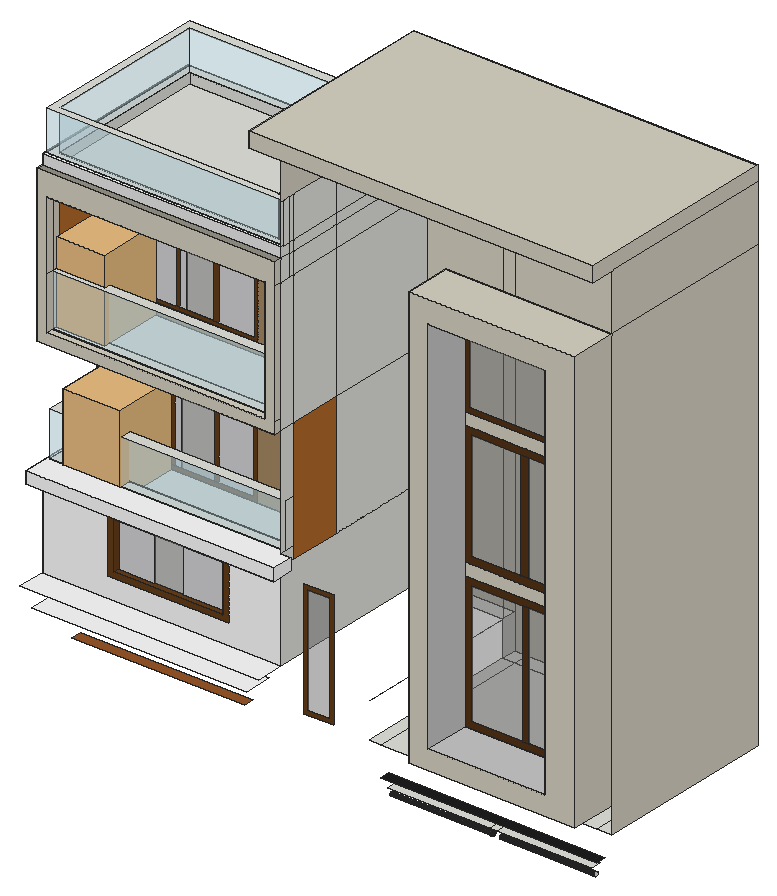
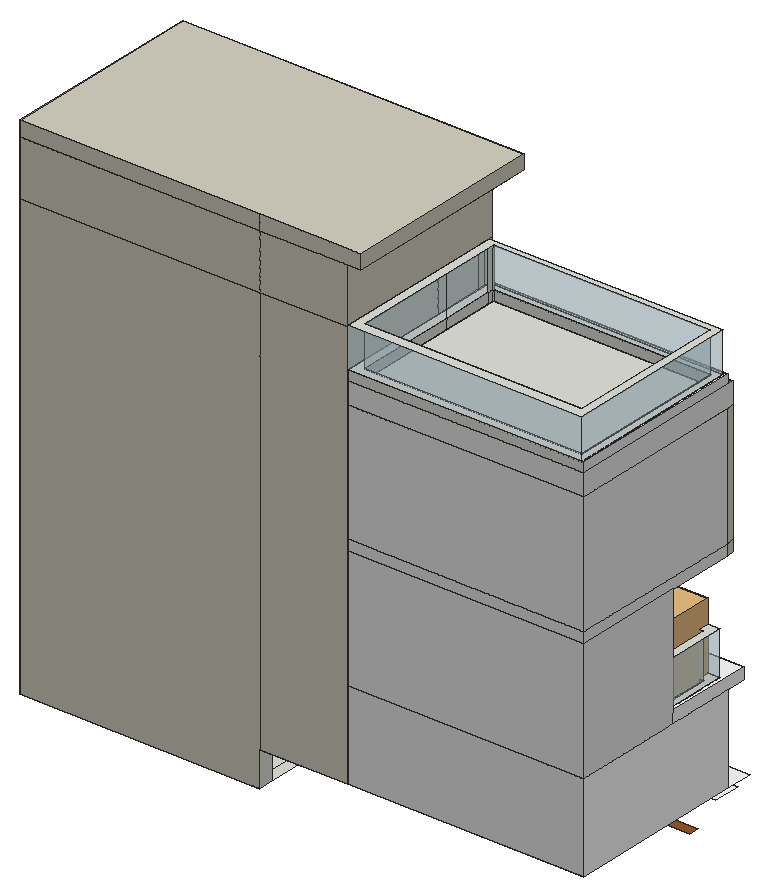
# SketchUp Ruby script. Lengths in inches.
U = 1.inch
M = Sketchup.active_model
def pt(a) = Geom::Point3d.new(a.map { |v| v * U })
def face(e, loops, mat)
  f = e.add_face(loops[0].map { |a| pt(a) })
  loops[1..].each { |l| e.add_face(l.map { |a| pt(a) }).erase! }
  f.material = f.back_material = mat if mat
  f
end
# faces: each face lists its corners as indices into pts; further lists are holes
def faces(e, pts, list, mat = nil) = list.each { |f| face(e, (f[0].is_a?(Array) ? f : [f]).map { |l| l.map { |i| pts[i] } }, mat) }
# xy, xz, yz: faces in a plane at the given z, y or x. An outline is a flat list of corners, or four numbers for a rectangle; further outlines are holes
def ring(l) = l.size == 4 ? [[l[0], l[1]], [l[2], l[1]], [l[2], l[3]], [l[0], l[3]]] : l.each_slice(2).to_a
def flat(e, list, mat, &to3) = list.each { |f| face(e, (f[0].is_a?(Array) ? f : [f]).map { |l| ring(l).map { |u, v| to3.(u, v) } }, mat) }
def xy(e, z, list, mat = nil) = flat(e, list, mat) { |x, y| [x, y, z] }
def xz(e, y, list, mat = nil) = flat(e, list, mat) { |x, z| [x, y, z] }
def yz(e, x, list, mat = nil) = flat(e, list, mat) { |y, z| [x, y, z] }
def lines(e, pts, list) = list.each { |a, b| e.add_line(pt(pts[a]), pt(pts[b])) }
# prism: a flat outline (further loops are holes) pulled along v
def prism(e, loops, v, mat = nil)
  f = face(e, loops, mat); d = Geom::Vector3d.new(v.map { |x| x * U })
  f.pushpull(f.normal.samedirection?(d) ? d.length : -d.length)
end
def box(e, o, s, mat = nil) = prism(e, [[o, [o[0] + s[0], o[1], o[2]], [o[0] + s[0], o[1] + s[1], o[2]], [o[0], o[1] + s[1], o[2]]]], [0, 0, s[2]], mat)
def at(x, y, z, deg = 0) = Geom::Transformation.translation(pt([x, y, z])) * Geom::Transformation.rotation(ORIGIN, Z_AXIS, deg.degrees)
def axes(o, x, y, z) = Geom::Transformation.new([*x, 0, *y, 0, *z, 0, *pt(o).to_a, 1])
def part(name) = M.definitions.add(name)
# library, detail: a bought-in or finely detailed component or shape, given as its bounding box
def library(name, o, s) = part(name).tap { |d| box(d.entities, o, s) }
def detail(e, o, s) = box(e.add_group.entities, o, s)
def put(e, d, t, mat = nil) = e.add_instance(d, t).tap { |i| i.material = mat if mat }
def group(e, t, mat = nil) = e.add_group.tap { |g| g.transformation = t; g.material = mat if mat }.entities
root = M.entities
M.materials.add("[Blinds Vertical Pattern]").color = [212, 212, 214]
M.materials.add("[Blinds Weave]").color = [141, 91, 25]
M.materials.add("[Carrera Marble]").color = [252, 252, 252]
M.materials.add("[Carrera Marble]1").color = [234, 234, 234]
M.materials.add("[Color M02]").color = [198, 198, 198]
M.materials.add("[Color M07]").color = [58, 58, 58]
M.materials.add("[Color M08]").color = [30, 30, 30]
M.materials.add("[Formica Graystone]").color = [214, 209, 194]
M.materials.add("[Formica Graystone]1").color = [149, 146, 135]
M.materials.add("[Quartz Light Grey]").color = [251, 251, 252]
M.materials.add("[Translucent Glass Gray]").color = [128, 128, 128]
M.materials["[Translucent Glass Gray]"].alpha = 0.5
M.materials.add("[Translucent Glass Safety]").color = [213, 245, 255]
M.materials["[Translucent Glass Safety]"].alpha = 0.35
M.materials.add("[Wallpaper Stripe]").color = [165, 138, 99]
M.materials.add("[Wood Bamboo]").color = [177, 105, 43]
M.materials.add("[Wood Cherry Original]").color = [152, 86, 42]
M.materials.add("[Wood Floor Dark]").color = [84, 51, 23]
M.materials.add("[Wood Floor Parquet]").color = [102, 62, 27]
M.materials.add("[Wood Floor Parquet]1").color = [145, 89, 39]
c1 = library("chau cay",[-24.34,-109.24,0],[56.46,62.58,79.69])
xy(root,113.6,[[473.77,406.29,574.36,416.16],[574.36,406.29,581.54,416.16],[581.54,406.29,674.94,416.16]])
xy(root,119.75,[[467.61,406.29,674.94,416.16],[674.94,406.29,679.23,416.16]],"[Color M08]")
xy(root,136.93,[[163.95,406.29,333.85,416.16]],"[Wood Cherry Original]")
xy(root,149.125,[[456.06,406.29,467.61,570.65],[467.61,406.29,679.23,570.65],[679.23,406.29,694.52,585.18],[456.06,570.65,467.61,585.18],[467.61,570.65,679.23,585.18]])
xy(root,168.73,[[146.33,378.85,357.05,406.29]],"[Carrera Marble]")
xy(root,175.14,[[531.06,361.1,694.52,406.29]],"[Formica Graystone]")
xy(root,183.6875,[[134.55,406.29,369,570.65],[134.55,570.65,369,585.18],[369,570.65,456.06,585.18]])
xy(root,183.6875,[[134.55,378.85,369,406.29]],"[Carrera Marble]")
xy(root,194.17,[[550.09,361.1,664.36,406.29]],"[Color M02]")
xy(root,208.41,[[204.29,406.29,312.26,412.54]],"[Wood Floor Parquet]")
xy(root,255.64,[[204.29,406.29,312.26,412.54]],"[Wood Floor Parquet]")
xy(root,270.8125,[[134.55,406.29,134.55,473.7,145.55,473.7,145.55,422.06,369,422.06,369,406.29],[145.55,422.06,369,473.7],[134.55,473.7,369,585.18]])
xy(root,270.8125,[[134.55,385.54,378.87,406.29]],"[Wood Bamboo]")
xy(root,276.39,[[320.76,473.7,360.82,482.32]],"[Wood Floor Parquet]1")
xy(root,282.625,[[137.78,411.51,137.78,473.7,145.55,473.7,145.55,422.06,369,422.06,369,411.51]])
xy(root,282.625,[[134.55,385.54,378.87,385.54,378.87,406.29,369,406.29,369,411.51,137.78,411.51,137.78,473.7,134.55,473.7]],"[Carrera Marble]")
xy(root,326.4375,[[137.78,411.51,369,411.51,369,422.06,145.55,422.06,145.55,473.7,137.78,473.7]])
xy(root,353.33,[[320.76,473.7,360.82,482.32]],"[Wood Floor Parquet]1")
xy(root,390.8125,[[134.55,406.29,145.55,473.7],[145.55,406.29,369,473.7],[134.55,473.7,369,585.18]])
xy(root,390.8125,[[134.55,399.16,145.55,406.29],[145.55,399.16,369,406.29]],"[Formica Graystone]")
xy(root,401.5,[[144.33,406.29,359.22,416.07],[144.33,416.07,359.22,473.7],[144.33,473.7,359.22,575.4]])
xy(root,401.5,[[144.33,399.16,359.22,406.29]],"[Formica Graystone]")
xy(root,416.25,[[308.63,473.7,346.63,482.95]])
xy(root,453.125,[[144.33,406.29,359.22,416.07]])
xy(root,483.25,[[308.63,473.7,346.63,482.95]],"[Wood Floor Parquet]1")
xy(root,521.5,[[134.55,406.29,144.33,416.07],[359.22,406.29,369,416.07],[134.55,416.07,144.33,473.7],[359.22,416.07,369,422.06],[359.22,422.06,369,473.7],
  [134.55,473.7,144.33,585.18],[144.33,473.7,359.22,575.4],[359.22,473.7,369,585.18],[144.33,575.4,359.22,585.18]])
xy(root,521.5,[[144.33,399.16,359.22,473.7]],"[Wood Bamboo]")
xy(root,542.8125,[[[134.55,406.29,369,585.18],[143.9,415.64,359.65,575.83]],[143.9,415.64,359.65,575.83]])
xy(root,542.8125,[[134.55,399.16,369,406.29]],"[Formica Graystone]1")
xy(root,552.5,[[[136.62,409.6,369,585.18],[143.9,415.64,359.65,575.83]]])
xy(root,552.5,[[134.55,406.29,369,409.6],[134.55,409.6,136.62,585.18]],"[Quartz Light Grey]")
xy(root,568.18,[[550.09,361.1,664.36,406.29]],"[Color M02]")
xy(root,590.25,[[531.06,361.1,694.52,406.29]],"[Formica Graystone]")
xy(root,592.1875,[[[136.62,409.6,369,585.18],[143.9,415.64,359.65,575.83]]])
xy(root,645.75,[[369,406.29,694.52,585.18]])
xy(root,645.75,[[356.12,382.85,694.52,406.29],[356.12,406.29,369,585.18]],"[Formica Graystone]")
xy(root,660.4375,[[356.12,382.85,694.52,585.18]],"[Formica Graystone]")
xz(root,361.1,[[[531.06,175.14,694.52,590.25],[550.09,194.17,664.36,568.18]]],"[Formica Graystone]")
xz(root,382.85,[[356.12,645.75,694.52,660.4375]],"[Formica Graystone]")
xz(root,385.54,[[134.55,270.8125,378.87,282.625]],"[Carrera Marble]")
xz(root,399.16,[[[134.55,390.8125,369,542.8125],[144.33,401.5,359.22,521.5]]],"[Formica Graystone]")
xz(root,406.29,[[[531.06,175.14,694.52,590.25],[550.09,194.17,664.36,568.18]],[369,270.8125,378.87,282.625],[134.55,390.8125,134.55,521.5,144.33,521.5,144.33,401.5,359.22,401.5,359.22,521.5,369,521.5,369,390.8125]])
xz(root,406.29,[[[134.55,183.6875,369,270.8125],[199.09,203.21,317.46,260.84]]],"[Carrera Marble]")
xz(root,406.29,[[134.55,542.8125,369,552.5]],"[Carrera Marble]1")
xz(root,406.29,[[550.09,326.9,664.36,339.04],[550.09,459.62,664.36,471.47]],"[Formica Graystone]")
xz(root,406.29,[[395.5625,153.71,416.96,260.54],[556.47,200.55,606.76,320.52],[612.79,200.55,657.99,320.52],[556.8,345.75,604.91,452.91],[612.27,345.75,657.65,452.91],
  [555.11,476.49,659.35,563.16]],"[Translucent Glass Gray]")
xz(root,406.29,[[144.33,401.5,359.22,453.125]],"[Translucent Glass Safety]")
xz(root,406.29,[[[550.09,194.17,664.36,326.9],[556.47,200.55,657.99,320.52]],[606.76,200.55,612.79,320.52],[[550.09,339.04,664.36,459.62],[556.8,345.75,657.65,452.91]],[604.91,345.75,612.27,452.91],[[550.09,471.47,664.36,568.18],[555.11,476.49,659.35,563.16]]],"[Wood Floor Dark]")
xz(root,406.29,[[[391.83,149.97,420.7,264.27],[395.5625,153.71,416.96,260.54]],[[199.09,203.21,317.46,260.84],[204.29,208.41,312.26,255.64]]],"[Wood Floor Parquet]")
xz(root,409.6,[[136.62,552.5,369,592.1875]],"[Translucent Glass Safety]")
xz(root,411.51,[[137.78,282.625,369,326.4375]],"[Translucent Glass Safety]")
xz(root,412.54,[[204.29,208.41,240,255.64],[268.36,208.41,312.26,255.64]],"[Blinds Vertical Pattern]")
xz(root,412.54,[[240,208.41,268.36,255.64]],"[Translucent Glass Gray]")
xz(root,415.64,[[143.9,542.8125,359.65,552.5]])
xz(root,415.64,[[143.9,552.5,359.65,592.1875]],"[Translucent Glass Safety]")
xz(root,416.07,[[144.33,401.5,359.22,453.125]],"[Translucent Glass Safety]")
xz(root,422.06,[[145.55,270.8125,369,282.625]])
xz(root,422.06,[[145.55,282.625,369,326.4375]],"[Translucent Glass Safety]")
xz(root,473.7,[[134.55,270.8125,145.55,282.625],[134.55,282.625,137.78,282.625,137.78,326.4375,145.55,326.4375,145.55,390.8125,134.55,390.8125],[137.78,282.625,145.55,326.4375]])
xz(root,473.7,[[175.44,274.72,207.12,374.1],[210.96,274.72,218.06,374.1],[254.34,274.72,288.69,374.1],[174.75,416.21,211.53,501.07],[216.17,416.21,223.04,501.07],
  [254.11,416.21,288.86,501.07]],"[Blinds Vertical Pattern]")
xz(root,473.7,[[218.06,274.72,250.5,374.1],[223.04,416.21,249.47,501.07]],"[Translucent Glass Gray]")
xz(root,473.7,[[[145.55,270.8125,171.54,270.8125,171.54,378,292.6,378,292.6,270.8125,369,270.8125,369,390.8125,145.55,390.8125],[320.76,276.39,360.82,353.33]],[[144.33,401.5,359.22,521.5],[170.84,412.3,292.77,504.98],[308.63,416.25,346.63,483.25]]],"[Wallpaper Stripe]")
xz(root,473.7,[[[171.54,270.8125,292.6,378],[175.44,274.72,288.69,374.1]],[207.12,274.72,210.96,374.1],[250.5,274.72,254.34,374.1],[[170.84,412.3,292.77,504.98],[174.75,416.21,288.86,501.07]],[211.53,416.21,216.17,501.07],
  [249.47,416.21,254.11,501.07]],"[Wood Floor Parquet]")
xz(root,482.32,[[320.76,276.39,360.82,353.33]],"[Blinds Weave]")
xz(root,482.95,[[308.63,416.25,346.63,483.25]],"[Blinds Weave]")
xz(root,575.4,[[144.33,401.5,359.22,521.5]])
xz(root,575.83,[[143.9,542.8125,359.65,552.5]])
xz(root,575.83,[[143.9,552.5,359.65,592.1875]],"[Translucent Glass Safety]")
xz(root,585.18,[[134.55,542.8125,369,552.5]])
xz(root,585.18,[[134.55,183.6875,369,270.8125],[134.55,270.8125,369,390.8125],[134.55,390.8125,369,401.5],[134.55,401.5,369,521.5],[134.55,521.5,369,542.8125]],"[Carrera Marble]1")
xz(root,585.18,[[456.06,149.125,694.52,590.25],[369,183.6875,456.06,590.25],[369,590.25,456.06,645.75],[456.06,590.25,694.52,645.75],[356.12,645.75,456.06,660.4375],
  [456.06,645.75,694.52,660.4375]],"[Formica Graystone]")
xz(root,585.18,[[136.62,552.5,369,592.1875]],"[Translucent Glass Safety]")
yz(root,134.55,[[406.29,183.6875,585.18,270.8125],[385.54,270.8125,473.7,282.625]],"[Carrera Marble]")
yz(root,134.55,[[473.7,270.8125,585.18,390.8125],[406.29,390.8125,585.18,401.5],[406.29,401.5,585.18,521.5],[399.16,521.5,585.18,542.8125],[406.29,542.8125,585.18,552.5]],"[Carrera Marble]1")
yz(root,134.55,[[399.16,390.8125,406.29,401.5],[399.16,401.5,406.29,521.5]],"[Formica Graystone]")
yz(root,136.62,[[409.6,552.5,585.18,592.1875]],"[Translucent Glass Safety]")
yz(root,137.78,[[411.51,282.625,473.7,326.4375]],"[Translucent Glass Safety]")
yz(root,143.9,[[415.64,542.8125,575.83,552.5]])
yz(root,143.9,[[415.64,552.5,575.83,592.1875]],"[Translucent Glass Safety]")
yz(root,144.33,[[406.29,401.5,416.07,453.125],[473.7,401.5,575.4,521.5]])
yz(root,144.33,[[399.16,401.5,406.29,453.125],[399.16,453.125,406.29,521.5],[406.29,453.125,416.07,521.5]],"[Formica Graystone]")
yz(root,144.33,[[416.07,401.5,473.7,521.5]],"[Wood Bamboo]")
yz(root,145.55,[[422.06,270.8125,473.7,282.625]])
yz(root,145.55,[[422.06,282.625,473.7,326.4375]],"[Translucent Glass Safety]")
yz(root,204.29,[[406.29,208.41,412.54,255.64]],"[Wood Floor Parquet]")
yz(root,308.63,[[473.7,416.25,482.95,483.25]],"[Wood Floor Parquet]1")
yz(root,312.26,[[406.29,208.41,412.54,255.64]],"[Wood Floor Parquet]")
yz(root,320.76,[[473.7,276.39,482.32,353.33]],"[Wood Floor Parquet]1")
yz(root,346.63,[[473.7,416.25,482.95,483.25]],"[Wood Floor Parquet]1")
yz(root,356.12,[[382.85,645.75,585.18,660.4375]],"[Formica Graystone]")
yz(root,359.22,[[406.29,401.5,416.07,453.125],[473.7,401.5,575.4,521.5]])
yz(root,359.22,[[399.16,401.5,406.29,453.125],[399.16,453.125,406.29,521.5],[406.29,453.125,416.07,521.5]],"[Formica Graystone]")
yz(root,359.22,[[416.07,401.5,422.06,521.5],[422.06,401.5,473.7,521.5]],"[Wood Bamboo]")
yz(root,359.65,[[415.64,542.8125,416.07,552.5],[416.07,542.8125,422.06,552.5],[422.06,542.8125,473.7,552.5],[473.7,542.8125,575.83,552.5],[415.64,552.5,416.07,592.1875],
  [416.07,552.5,422.06,592.1875]])
yz(root,359.65,[[422.06,552.5,473.7,592.1875],[473.7,552.5,575.83,592.1875]],"[Translucent Glass Safety]")
yz(root,360.82,[[473.7,276.39,482.32,353.33]],"[Wood Floor Parquet]1")
yz(root,369,[[406.29,183.6875,585.18,270.8125],[406.29,270.8125,422.06,282.625],[473.7,270.8125,585.18,390.8125],[406.29,282.625,406.29,390.8125,422.06,390.8125,422.06,326.4375,411.51,326.4375,411.51,282.625],[411.51,282.625,422.06,326.4375],
  [406.29,390.8125,422.06,521.5],[422.06,390.8125,473.7,521.5],[473.7,390.8125,585.18,521.5],[406.29,521.5,416.07,542.8125],[416.07,521.5,422.06,542.8125],
  [422.06,521.5,473.7,542.8125],[473.7,521.5,585.18,542.8125],[406.29,542.8125,416.07,552.5],[416.07,542.8125,422.06,552.5],[422.06,542.8125,473.7,552.5],
  [473.7,542.8125,585.18,552.5],[406.29,552.5,409.6,592.1875],[409.6,552.5,416.07,592.1875],[416.07,552.5,422.06,592.1875],[422.06,552.5,473.7,592.1875],
  [473.7,552.5,585.18,592.1875]])
yz(root,369,[[399.16,390.8125,406.29,401.5],[399.16,401.5,406.29,521.5],[399.16,521.5,406.29,542.8125],[406.29,592.1875,585.18,645.75]],"[Formica Graystone]")
yz(root,369,[[422.06,270.8125,473.7,390.8125]],"[Wood Bamboo]")
yz(root,378.87,[[385.54,270.8125,406.29,282.625]],"[Carrera Marble]")
yz(root,456.06,[[570.65,149.125,585.18,183.6875]])
yz(root,473.77,[[411.5,103.75,411,103.8125,410.53,104.01,410.13,104.32,409.82,104.72,409.63,105.18,409.5625,105.6875,409.63,106.1875,409.82,106.65,410.13,107.06,410.53,107.36,411,107.56,411.5,107.625,412,107.56,412.47,107.36,412.87,107.06,413.18,106.65,413.37,106.1875,413.4375,105.6875,413.37,105.18,413.18,104.72,412.87,104.32,412.47,104.01,412,103.8125]])
yz(root,531.06,[[361.1,175.14,406.29,590.25]],"[Formica Graystone]")
yz(root,550.09,[[361.1,194.17,406.29,568.18]],"[Color M02]")
yz(root,664.36,[[361.1,194.17,406.29,568.18]],"[Color M02]")
yz(root,674.94,[[411.43,103.83,411.93,103.9,412.39,104.09,412.8,104.4,413.1,104.8,413.3,105.27,413.36,105.77,413.3,106.27,413.1,106.74,412.8,107.14,412.39,107.45,411.93,107.64,411.43,107.71,410.92,107.64,410.46,107.45,410.06,107.14,409.75,106.74,409.55,106.27,409.49,105.77,409.55,105.27,409.75,104.8,410.06,104.4,410.46,104.09,410.92,103.9]])
yz(root,694.52,[[406.29,149.125,585.18,590.25],[361.1,175.14,406.29,590.25],[406.29,590.25,585.18,645.75],[382.85,645.75,585.18,660.4375]],"[Formica Graystone]")
p = [[473.77,411,103.8125],[473.77,411.5,103.75],[574.36,411.5,103.75],[574.36,411,103.8125],[473.77,412,103.8125],[574.36,412,103.8125],
  [473.77,410.53,104.01],[574.36,410.53,104.01],[674.94,411.43,103.83],[674.94,410.92,103.9],[581.54,410.92,103.9],[581.54,411.43,103.83],
  [674.94,411.93,103.9],[581.54,411.93,103.9],[473.77,412.47,104.01],[574.36,412.47,104.01],[674.94,410.46,104.09],[581.54,410.46,104.09],
  [674.94,412.39,104.09],[581.54,412.39,104.09],[473.77,410.13,104.32],[574.36,410.13,104.32],[473.77,412.87,104.32],[574.36,412.87,104.32],
  [674.94,410.06,104.4],[581.54,410.06,104.4],[674.94,412.8,104.4],[581.54,412.8,104.4],[473.77,409.82,104.72],[574.36,409.82,104.72],
  [473.77,413.18,104.72],[574.36,413.18,104.72],[674.94,409.75,104.8],[581.54,409.75,104.8],[674.94,413.1,104.8],[581.54,413.1,104.8],
  [473.77,409.63,105.18],[574.36,409.63,105.18],[473.77,413.37,105.18],[574.36,413.37,105.18],[674.94,409.55,105.27],[581.54,409.55,105.27],
  [674.94,413.3,105.27],[581.54,413.3,105.27],[473.77,409.5625,105.6875],[574.36,409.5625,105.6875],[473.77,413.4375,105.6875],[574.36,413.4375,105.6875],
  [674.94,409.49,105.77],[581.54,409.49,105.77],[674.94,413.36,105.77],[581.54,413.36,105.77],[473.77,409.63,106.1875],[574.36,409.63,106.1875],
  [473.77,413.37,106.1875],[574.36,413.37,106.1875],[674.94,409.55,106.27],[581.54,409.55,106.27],[674.94,413.3,106.27],[581.54,413.3,106.27],
  [473.77,409.82,106.65],[574.36,409.82,106.65],[473.77,413.18,106.65],[574.36,413.18,106.65],[674.94,409.75,106.74],[581.54,409.75,106.74],
  [674.94,413.1,106.74],[581.54,413.1,106.74],[674.94,410.06,107.14],[581.54,410.06,107.14],[473.77,410.13,107.06],[574.36,410.13,107.06],
  [674.94,412.8,107.14],[581.54,412.8,107.14],[473.77,412.87,107.06],[574.36,412.87,107.06],[473.77,410.53,107.36],[574.36,410.53,107.36],
  [674.94,410.46,107.45],[581.54,410.46,107.45],[674.94,412.39,107.45],[581.54,412.39,107.45],[473.77,412.47,107.36],[574.36,412.47,107.36],
  [473.77,411,107.56],[574.36,411,107.56],[674.94,410.92,107.64],[581.54,410.92,107.64],[674.94,411.93,107.64],[581.54,411.93,107.64],
  [473.77,412,107.56],[574.36,412,107.56],[674.94,411.43,107.71],[581.54,411.43,107.71],[473.77,411.5,107.625],[574.36,411.5,107.625],
  [456.06,570.65,183.6875],[456.06,570.65,529.125],[456.06,406.29,183.6875]]
faces(root,p,[[0,1,2,3],[1,4,5,2],[6,0,3,7],[8,9,10,11],[12,8,11,13],[4,14,15,5],[9,16,17,10],[18,12,13,19],
  [20,6,7,21],[14,22,23,15],[16,24,25,17],[26,18,19,27],[28,20,21,29],[22,30,31,23],[24,32,33,25],[34,26,27,35],
  [36,28,29,37],[30,38,39,31],[32,40,41,33],[42,34,35,43],[44,36,37,45],[38,46,47,39],[40,48,49,41],[50,42,43,51],
  [52,44,45,53],[46,54,55,47],[48,56,57,49],[58,50,51,59],[60,52,53,61],[54,62,63,55],[56,64,65,57],[66,58,59,67],
  [64,68,69,65],[70,60,61,71],[72,66,67,73],[62,74,75,63],[76,70,71,77],[68,78,79,69],[80,72,73,81],[74,82,83,75],
  [84,76,77,85],[78,86,87,79],[88,80,81,89],[82,90,91,83],[86,92,93,87],[94,84,85,95],[92,88,89,93],[90,94,95,91]],"[Color M07]")
lines(root,p,[[96,97],[96,98]])
put(root,c1,at(175,520.35,269.57))
put(root,c1,at(160.26,520.35,401.5))
